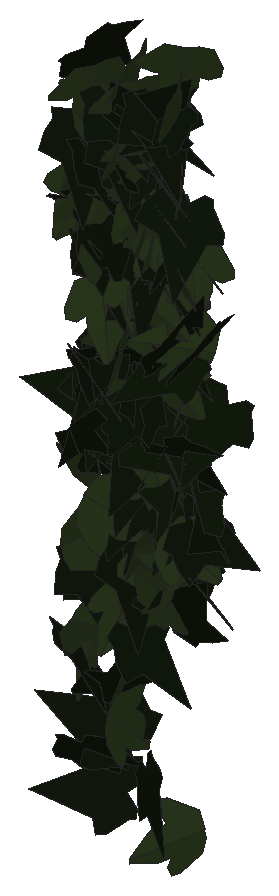
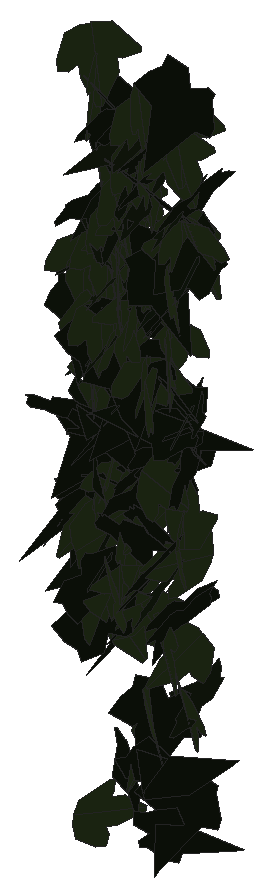
# SketchUp Ruby script. Lengths in inches.
U = 1.inch
M = Sketchup.active_model
def pt(a) = Geom::Point3d.new(a.map { |v| v * U })
def face(e, loops, mat)
  f = e.add_face(loops[0].map { |a| pt(a) })
  loops[1..].each { |l| e.add_face(l.map { |a| pt(a) }).erase! }
  f.material = f.back_material = mat if mat
  f
end
# faces: each face lists its corners as indices into pts; further lists are holes
def faces(e, pts, list, mat = nil) = list.each { |f| face(e, (f[0].is_a?(Array) ? f : [f]).map { |l| l.map { |i| pts[i] } }, mat) }
# xy, xz, yz: faces in a plane at the given z, y or x. An outline is a flat list of corners, or four numbers for a rectangle; further outlines are holes
def ring(l) = l.size == 4 ? [[l[0], l[1]], [l[2], l[1]], [l[2], l[3]], [l[0], l[3]]] : l.each_slice(2).to_a
def flat(e, list, mat, &to3) = list.each { |f| face(e, (f[0].is_a?(Array) ? f : [f]).map { |l| ring(l).map { |u, v| to3.(u, v) } }, mat) }
def xy(e, z, list, mat = nil) = flat(e, list, mat) { |x, y| [x, y, z] }
def xz(e, y, list, mat = nil) = flat(e, list, mat) { |x, z| [x, y, z] }
def yz(e, x, list, mat = nil) = flat(e, list, mat) { |y, z| [x, y, z] }
def lines(e, pts, list) = list.each { |a, b| e.add_line(pt(pts[a]), pt(pts[b])) }
# prism: a flat outline (further loops are holes) pulled along v
def prism(e, loops, v, mat = nil)
  f = face(e, loops, mat); d = Geom::Vector3d.new(v.map { |x| x * U })
  f.pushpull(f.normal.samedirection?(d) ? d.length : -d.length)
end
def box(e, o, s, mat = nil) = prism(e, [[o, [o[0] + s[0], o[1], o[2]], [o[0] + s[0], o[1] + s[1], o[2]], [o[0], o[1] + s[1], o[2]]]], [0, 0, s[2]], mat)
def at(x, y, z, deg = 0) = Geom::Transformation.translation(pt([x, y, z])) * Geom::Transformation.rotation(ORIGIN, Z_AXIS, deg.degrees)
def axes(o, x, y, z) = Geom::Transformation.new([*x, 0, *y, 0, *z, 0, *pt(o).to_a, 1])
def part(name) = M.definitions.add(name)
# library, detail: a bought-in or finely detailed component or shape, given as its bounding box
def library(name, o, s) = part(name).tap { |d| box(d.entities, o, s) }
def detail(e, o, s) = box(e.add_group.entities, o, s)
def put(e, d, t, mat = nil) = e.add_instance(d, t).tap { |i| i.material = mat if mat }
def group(e, t, mat = nil) = e.add_group.tap { |g| g.transformation = t; g.material = mat if mat }.entities
root = M.entities
M.materials.add("efeu1").color = [18, 25, 13]
M.materials.add("efeu2").color = [43, 57, 29]
c1 = part("ivyleaf_10")
p = [[0,0.5,-0.03],[-0.0625,2.02,-0.43],[-0.19,2.01,-0.46],[-0.54,1.05,-0.29],[-0.52,0.625,-0.18],[-0.83,0.76,-0.28],
  [-1.16,0.64,-0.33],[-1.15,0.33,-0.24],[-0.77,-0.39,0.02],[-0.3,-0.51,0.16],[0.04,-0.48,0.23],[-0.02,2.01,-0.4375],
  [-0.06,2.01,-0.43],[0.04,-0.49,0.23],[0.67,-0.49,0.14],[1.38,0.36,-0.2],[1.375,0.51,-0.24],[0.81,0.65,-0.19],
  [0.62,0.59,-0.15],[0.6,1.09,-0.28],[0.5,1.23,-0.31]]
faces(c1.entities,p,[[0,1,2,3,4,5,6,7,8,9,10],[11,12,0,13,14,15,16,17,18,19,20]],"efeu2")
c2 = part("ivyleaf_9")
p = [[1.54,2.16,1.25],[1.36,2.04,1.19],[-0.21,0.99,0.68],[-0.71,1.11,0.82],[-0.85,0.86,0.67],[-0.8,0.17,0.21],
  [-0.9,-0.01,0.1],[-0.67,-0.16,-0.02],[-0.08,-0.08,-0.05],[-0.03,-0.6,-0.4],[0.65,-0.88,-0.66],[0.83,-0.6,-0.49],
  [1.29,-0.42,-0.43],[1.8125,-0.07,-0.26],[1.21,0.44,0.15]]
faces(c2.entities,p,[[0,1,2,3,4,5,6,7,8,9,10,11,12,13,14]],"efeu1")
put(root,c1,axes([534.62,135.42,188.35],[0.65935,-0.44061,0.12588],[0.1096,-0.06254,-0.79297],[0.44494,0.66834,0.00879]))
put(root,c1,axes([534.84,134.72,201.15],[0.75412,-0.21779,-0.249],[-0.2252,0.11603,-0.78355],[0.24231,0.78564,0.04669]))
put(root,c2,axes([534.76,135.05,185.55],[0.67039,0.39495,-0.20021],[-0.17138,-0.10353,-0.77808],[-0.40829,0.69195,-0.00214]))
put(root,c2,axes([534.37,135.18,188.14],[0.29214,-0.6095,0.36994],[0.24797,-0.28798,-0.67028],[0.66848,0.37319,0.08696]))
put(root,c2,axes([535.5,135.61,184.25],[-0.50673,-0.01581,0.6028],[-0.60281,-0.00682,-0.50692],[0.01539,-0.78746,-0.00771]))
put(root,c2,axes([535.57,134.98,195.46],[-0.46793,0.18813,0.62786],[-0.63373,0.06703,-0.49239],[-0.16728,-0.78018,0.1091]))
put(root,c2,axes([534.68,135.07,202.5],[0.04718,-0.829,0.02894],[-0.02015,-0.03012,-0.83005],[0.82926,0.04644,-0.02181]))
put(root,c2,axes([535.57,135.64,185.74],[-0.16714,0.06845,0.8358],[-0.83569,0.05731,-0.17181],[-0.06977,-0.85042,0.0557]))
put(root,c1,axes([535.02,135.42,200.09],[0.28756,-0.76041,-0.04757],[-0.01021,0.04699,-0.81294],[0.76183,0.28765,0.00706]))
put(root,c1,axes([534.85,135.1,192.89],[-0.73914,0.10485,0.29304],[0.28257,-0.09043,0.74509],[0.13045,0.78995,0.0464]))
put(root,c1,axes([535.38,135.08,203.71],[-0.68667,-0.27736,0.36474],[-0.30278,-0.21857,-0.73623],[0.34393,-0.74618,0.08008]))
put(root,c2,axes([534.64,134.71,200.8125],[0.78179,0.14935,0.20417],[0.16207,0.21347,-0.77675],[-0.19422,0.7793,0.17365]))
put(root,c2,axes([534.8,135.32,194.78],[0.10445,-0.27062,-0.74441],[0.57646,-0.48897,0.25864],[-0.54321,-0.57094,0.13134]))
put(root,c2,axes([534.85,134.99,196.34],[0.56446,-0.45809,-0.33124],[-0.257,0.20897,-0.72696],[0.50351,0.62021,0.00028]))
put(root,c1,axes([535.4,135.1,197.8],[0.17744,-0.38074,-0.71286],[-0.30426,0.64467,-0.42006],[0.7487,0.35221,-0.00176]))
put(root,c1,axes([535.18,136,194.66],[-0.01205,-0.56281,0.54498],[0.03984,-0.54478,-0.56172],[0.78241,0.01907,0.03699]))
put(root,c1,axes([534.75,135.48,192.54],[0.21381,-0.30403,0.73736],[0.5785,-0.46643,-0.36006],[0.54907,0.60981,0.09223]))
put(root,c2,axes([534.86,135.24,190.64],[0.22126,-0.70973,-0.26985],[-0.06169,0.26334,-0.7432],[0.75679,0.22897,0.01831]))
put(root,c2,axes([535.15,134.67,205.17],[0.31691,0.72566,0.23951],[0.12455,0.20678,-0.79127],[-0.75395,0.33918,-0.03004]))
put(root,c1,axes([535.1875,134.81,201.23],[-0.1308,-0.81296,-0.08467],[0.09636,0.06981,-0.81916],[0.81166,-0.1393,0.08361]))
put(root,c1,axes([535.28,134.83,204.375],[-0.35242,-0.76911,-0.03582],[0.01252,0.03367,-0.846],[0.76984,-0.35264,-0.00264]))
put(root,c2,axes([534.95,135.07,190.81],[0.0908,-0.72471,-0.26389],[-0.02171,0.2632,-0.7303],[0.77095,0.09277,0.01051]))
put(root,c1,axes([535.18,134.71,201.09],[-0.80741,-0.01746,-0.16808],[0.16765,0.01997,-0.80745],[0.02116,-0.82448,-0.016]))
put(root,c2,axes([534.95,134.81,200.48],[0.67852,-0.34345,-0.31279],[-0.23656,0.22106,-0.75588],[0.39979,0.71369,0.08361]))
put(root,c2,axes([535.55,135.38,200.37],[-0.22617,0.73716,-0.26414],[0.01669,-0.27033,-0.76874],[-0.78287,-0.21873,0.05992]))
put(root,c2,axes([535.1875,135.68,195.46],[-0.32941,-0.71418,0.01216],[-0.00033,-0.01324,-0.78647],[0.71428,-0.32937,0.00525]))
put(root,c1,axes([535.09,134.57,189.33],[-0.2664,-0.34579,-0.60588],[0.35096,0.49407,-0.43629],[0.6029,-0.4404,-0.01374]))
put(root,c1,axes([535.19,134.3125,191.69],[0.0237,-0.15167,0.87928],[-0.02671,0.87908,0.15235],[-0.89187,-0.03036,0.0188]))
put(root,c1,axes([535.58,135.17,189.86],[0.50124,-0.42503,-0.47194],[-0.29702,0.37454,-0.65278],[0.56138,0.57766,0.076]))
put(root,c2,axes([534.85,135.25,195.66],[0.18346,-0.44461,0.62928],[0.37405,-0.51415,-0.47231],[0.67362,0.40658,0.09088]))
put(root,c2,axes([535.06,135.19,199.48],[0.3081,-0.73797,-0.06503],[-0.00691,0.06756,-0.79947],[0.7408,0.30756,0.01959]))
put(root,c2,axes([534.82,135.23,196.13],[0.55414,-0.133,0.56275],[0.5721,0.23954,-0.50673],[-0.08417,0.75258,0.26074]))
put(root,c2,axes([535.53,135.23,196.9375],[-0.70733,-0.01372,-0.3327],[0.33297,-0.03678,-0.70638],[-0.00326,-0.7808,0.03912]))
put(root,c2,axes([535.53,135.0625,187.78],[0.43921,0.647,-0.13895],[-0.0784,-0.11472,-0.78199],[-0.65709,0.44615,0.00042]))
put(root,c2,axes([535.2,135.88,192.2],[0.18454,-0.7603,0.01318],[0.00395,-0.0126,-0.78238],[0.76041,0.18458,0.00087]))
put(root,c2,axes([535.07,134.99,202],[0.46871,-0.68381,0.0131],[0.03688,0.00941,-0.82826],[0.68295,0.4688,0.03573]))
put(root,c1,axes([535.45,135.78,196.91],[0.28905,-0.69765,0.23424],[0.21192,-0.16209,-0.74428],[0.70475,0.33488,0.12773]))
put(root,c2,axes([535.2,135.68,191.3],[0.31404,-0.70545,0.17567],[0.06055,-0.16532,-0.7721],[0.72447,0.31961,-0.01162]))
put(root,c1,axes([535.68,135.51,187.83],[0.36324,-0.67557,-0.0886],[-0.05749,0.06965,-0.76684],[0.67893,0.36735,-0.01753]))
put(root,c1,axes([535.43,134.85,198.39],[0.79984,0.16606,0.22125],[0.21587,0.04862,-0.81689],[-0.17299,0.82845,0.00359]))
put(root,c1,axes([535.83,135.38,197.18],[-0.64268,-0.45043,0.00271],[-0.00221,-0.00157,-0.78481],[0.45043,-0.64269,0.00002]))
put(root,c1,axes([535.77,134.32,200.26],[0.06572,0.58553,0.60075],[-0.10493,0.6036,-0.57682],[-0.8323,-0.02987,0.12015]))
put(root,c1,axes([535.97,134.875,186.68],[-0.11002,0.53422,0.6029],[-0.18627,0.57514,-0.54361],[-0.7837,-0.21169,0.04457]))
put(root,c2,axes([535.36,134.42,194.16],[0.25036,-0.00027,0.79652],[0.77861,0.17616,-0.24467],[-0.16798,0.81615,0.05308]))
put(root,c1,axes([535.87,135.5,196.83],[-0.0549,0.31499,-0.746],[0.03855,-0.74585,-0.31776],[-0.80886,-0.05692,0.03549]))
put(root,c2,axes([535.9,134.56,199.56],[-0.19596,-0.34475,0.75162],[0.58761,0.48542,0.37585],[-0.58181,0.60638,0.12644]))
put(root,c2,axes([535.65,135.13,203.71],[0.2342,-0.74444,-0.2667],[0.0546,0.29271,-0.7691],[0.78889,0.20074,0.1324]))
put(root,c1,axes([536.13,135.04,190.14],[0.47574,0.52141,-0.33208],[-0.24723,-0.22359,-0.70524],[-0.56659,0.53536,0.02889]))
put(root,c1,axes([536.18,135.23,204.83],[0.17272,-0.79658,-0.11877],[-0.01567,0.11813,-0.81503],[0.80523,0.17316,0.00962]))
put(root,c1,axes([536.18,134.96,202.875],[0.19418,-0.7978,-0.16362],[-0.00479,0.16709,-0.82038],[0.81439,0.1912,0.03419]))
put(root,c2,axes([536.8,134.53,195.84],[-0.61517,0.45173,0.46743],[-0.37646,0.27706,-0.76321],[-0.52993,-0.72122,-0.00043]))
put(root,c2,axes([536.33,135.34,197.54],[0.44798,0.52469,-0.43253],[-0.35392,-0.26235,-0.68482],[-0.58062,0.56475,0.08372]))
put(root,c2,axes([536.3,135.27,192.99],[-0.7213,-0.06709,-0.23637],[0.23694,0.0041,-0.72421],[0.06504,-0.75903,0.01699]))
put(root,c2,axes([535.87,135.1,202.79],[0.16429,-0.81077,-0.06081],[-0.02385,0.05721,-0.82716],[0.8127,0.16558,-0.01198]))
put(root,c2,axes([536.81,135.09,202.33],[-0.67465,0.34949,0.34378],[-0.36781,0.02578,-0.74802],[-0.3241,-0.75676,0.13328]))
put(root,c2,axes([536.07,135.6875,193.91],[-0.24356,-0.75318,0.12948],[-0.02391,-0.12832,-0.7914],[0.76385,-0.24417,0.01651]))
put(root,c1,axes([535.97,134.14,193.01],[0.12189,0.57494,0.68034],[0.13848,0.6661,-0.58771],[-0.87991,0.18448,0.00175]))
put(root,c2,axes([535.97,135.1,196.61],[0.69878,0.39802,0.06626],[0.05292,0.04097,-0.80413],[-0.40001,0.70071,0.00938]))
put(root,c1,axes([536.4,134.99,204.26],[-0.3645,-0.74114,0.00565],[-0.00315,-0.00475,-0.82592],[0.74115,-0.36451,-0.00073]))
put(root,c2,axes([536.32,135.84,192.85],[-0.63495,-0.31036,-0.28574],[0.28803,0.05834,-0.70339],[0.30824,-0.69383,0.06867]))
put(root,c2,axes([536.24,135.4,194.29],[-0.13244,-0.68712,0.35712],[-0.07492,-0.34923,-0.69973],[0.77075,-0.15202,-0.00666]))
put(root,c1,axes([536.35,135.26,198.91],[-0.30631,0.64826,-0.3505],[-0.0139,-0.38458,-0.69916],[-0.73682,-0.26224,0.1589]))
put(root,c1,axes([536.27,135.28,198.92],[0.49155,0.62875,0.00723],[0.00104,0.00836,-0.79808],[-0.62879,0.49153,0.00433]))
put(root,c1,axes([536.58,135.08,202.99],[-0.14124,-0.81188,0.10003],[-0.02726,-0.09678,-0.82401],[0.81756,-0.14349,-0.01019]))
put(root,c2,axes([536.14,135.17,190.97],[0.12675,-0.77791,0.17103],[0.05606,-0.16404,-0.78766],[0.79451,0.13567,0.02829]))
put(root,c2,axes([536.02,135.18,202.03],[0.59458,-0.57068,0.06103],[0.10893,0.02594,-0.81878],[0.5635,0.59714,0.09388]))
put(root,c1,axes([536.44,135.1875,191.1],[0.2707,0.72972,0.18984],[0.06971,0.17662,-0.7783],[-0.75077,0.27951,-0.00382]))
put(root,c1,axes([536.74,135.22,202.02],[-0.25605,-0.78178,0.04635],[-0.00725,-0.0464,-0.82261],[0.78312,-0.25604,0.00754]))
put(root,c1,axes([536.67,135.17,200.75],[0.39345,-0.72155,-0.09482],[0.01599,0.11633,-0.81892],[0.72757,0.38763,0.06927]))
put(root,c1,axes([536.74,135.03,192.05],[0.12936,-0.71454,-0.36284],[0.00732,0.36857,-0.72323],[0.80136,0.11198,0.06518]))
put(root,c1,axes([537.08,135.46,190.1],[-0.51209,-0.35145,0.50491],[-0.3983,-0.31126,-0.62062],[0.46884,-0.6483,0.02425]))
put(root,c2,axes([536.54,134.98,196.08],[0.47358,-0.22128,-0.60084],[-0.28342,0.59768,-0.44351],[0.57415,0.47756,0.27666]))
put(root,c1,axes([536.67,134.77,201.24],[0.22358,0.77697,0.06202],[-0.03068,0.07325,-0.80698],[-0.77884,0.22016,0.0496]))
put(root,c1,axes([536.68,135.5,190.25],[0.59652,-0.54701,0.10178],[-0.05942,0.08573,0.80903],[-0.55322,-0.59904,0.02285]))
put(root,c2,axes([536.54,135.49,198.76],[-0.33373,-0.51834,-0.50701],[0.38098,0.34953,-0.60811],[0.61692,-0.49625,0.10126]))
put(root,c1,axes([536.96,135.37,199.86],[0.47548,-0.56022,-0.32375],[-0.14223,0.30144,-0.73051],[0.63122,0.48992,0.07927]))
put(root,c2,axes([536.39,135.02,203.68],[0.70682,-0.4366,-0.08092],[0.08441,0.28147,-0.78129],[0.43593,0.65339,0.28249]))
put(root,c2,axes([536.78,135.12,199.92],[-0.60141,-0.14342,-0.53726],[0.5297,0.09306,-0.61779],[0.16921,-0.80105,0.02442]))
put(root,c1,axes([536.85,135.36,198.08],[0.74408,-0.28657,-0.11983],[0.00017,0.31143,-0.74374],[0.31062,0.68631,0.28745]))
put(root,c1,axes([536.97,135.21,197.76],[-0.25013,0.76244,-0.04402],[-0.10858,-0.08136,-0.7921],[-0.75596,-0.24059,0.12833]))
put(root,c1,axes([536.8125,135.26,199.93],[0.33824,-0.71561,0.13946],[0.24483,-0.03333,-0.76479],[0.68673,0.36434,0.20396]))
put(root,c1,axes([537.12,135.46,190.25],[-0.26786,-0.50231,-0.56287],[-0.27471,-0.49135,0.56921],[-0.70262,0.3836,-0.00796]))
put(root,c1,axes([536.9,135.15,193.76],[-0.55826,-0.46717,-0.23901],[0.31045,-0.01268,-0.70034],[0.42307,-0.60714,0.19854]))
put(root,c1,axes([537.18,135.6,198.46],[-0.44689,-0.6571,0.00396],[-0.01023,0.00216,-0.79461],[0.65703,-0.4469,-0.00967]))
put(root,c1,axes([537.18,135.35,200.43],[-0.59415,-0.54419,-0.00207],[-0.00044,0.00355,-0.8057],[0.5442,-0.59415,-0.00291]))
put(root,c1,axes([537.16,135.18,201.08],[-0.21659,-0.79568,0.03401],[0.00997,-0.03795,-0.8244],[0.79634,-0.21593,0.01957]))
put(root,c2,axes([536.75,134.51,189.625],[0.44554,-0.55438,-0.39868],[-0.11042,0.41128,-0.6953],[0.67386,0.43393,0.14966]))
put(root,c2,axes([536.73,135.44,199.84],[0.43806,-0.68165,-0.06351],[0.01579,0.08544,-0.8081],[0.68442,0.43431,0.05929]))
put(root,c2,axes([537.34,136.05,191.17],[-0.012,-0.02168,-0.77136],[0.12578,-0.76119,0.01944],[-0.76135,-0.12541,0.01537]))
put(root,c2,axes([536.78,134.97,185.48],[-0.12587,-0.08121,-0.76685],[0.77097,-0.02924,-0.12345],[-0.01587,-0.77656,0.08484]))
put(root,c2,axes([536.8,134.79,203.44],[-0.27642,-0.1586,0.77641],[0.74387,-0.33539,0.19633],[0.27317,0.75282,0.25103]))
put(root,c2,axes([536.92,134.95,202.3125],[0.7595,-0.24942,-0.17916],[-0.16331,0.07673,-0.79912],[0.26008,0.77656,0.02141]))
put(root,c2,axes([537.67,134.96,200.37],[-0.54927,0.60141,-0.01408],[0.01065,-0.00935,-0.81448],[-0.60148,-0.54937,-0.00156]))
put(root,c1,axes([537.3,135.16,194.24],[-0.55741,0.54017,0.0108],[-0.00872,0.00652,-0.7762],[-0.54021,-0.55747,0.00139]))
put(root,c2,axes([536.89,135.41,197.97],[0.51506,-0.61224,-0.09127],[0.00715,0.12461,-0.79554],[0.61897,0.50802,0.08514]))
put(root,c1,axes([537.1875,135.16,200.22],[0.38768,0.70478,0.03202],[0.01904,0.02608,-0.80436],[-0.70525,0.38813,-0.00411]))
put(root,c2,axes([537.91,135.36,194.87],[-0.65386,-0.00067,0.41071],[-0.41046,-0.02625,-0.6535],[0.01453,-0.77171,0.02187]))
put(root,c2,axes([537.11,135.03,204.08],[0.0554,-0.78877,-0.26566],[-0.01652,0.26515,-0.79071],[0.83214,0.05777,0.00198]))
put(root,c1,axes([536.85,134.82,198.79],[-0.28131,-0.02452,-0.75855],[0.70365,-0.31156,-0.25088],[-0.28439,-0.74664,0.1296]))
put(root,c1,axes([537.17,135.2,196.69],[-0.68935,-0.16399,-0.41324],[0.41581,0.03205,-0.70636],[0.15736,-0.80309,0.0562]))
put(root,c2,axes([536.98,135.64,189.61],[0.82613,0.079,-0.10325],[0.08781,0.15072,0.8179],[0.09587,-0.8188,0.14059]))
put(root,c1,axes([537.71,135.48,191.77],[-0.12254,-0.1424,-0.78255],[-0.40287,-0.67159,0.1853],[-0.68582,0.41995,0.03097]))
put(root,c2,axes([537.94,134.92,204.41],[-0.78988,0.28737,0.03998],[-0.04529,-0.0076,-0.84022],[-0.28658,-0.79085,0.0226]))
put(root,c1,axes([537.69,135.4,183.92],[-0.16005,-0.02137,0.78363],[-0.12328,-0.78916,-0.0467],[0.77417,-0.13009,0.15457]))
put(root,c2,axes([537.98,135.05,197.48],[-0.765,-0.07871,0.18196],[-0.17628,-0.06188,-0.76787],[0.09073,-0.7839,0.04235]))
put(root,c2,axes([537.85,134.67,193.46],[-0.04655,0.20816,0.79895],[-0.06491,0.79682,-0.21138],[-0.82307,-0.07462,-0.02851]))
put(root,c2,axes([537.19,135.11,201.02],[0.74961,-0.31422,-0.06319],[-0.06123,0.01738,-0.81277],[0.31461,0.75207,-0.00762]))
put(root,c1,axes([537.55,135.08,202.34],[0.64081,-0.52438,0.07588],[0.13255,0.04337,-0.81971],[0.513,0.64383,0.11702]))
put(root,c1,axes([537.94,135,196.92],[0.25869,-0.50635,-0.65736],[-0.27444,0.5976,-0.56832],[0.78307,0.37672,0.01798]))
put(root,c2,axes([537.99,135.01,195.86],[-0.55514,0.56396,-0.37891],[0.24057,-0.29445,-0.79071],[-0.63542,-0.60419,0.03168]))
put(root,c2,axes([537.52,134.84,194.83],[0.70419,0.3322,0.01886],[0.0174,0.00732,-0.77862],[-0.33228,0.70441,-0.00081]))
put(root,c1,axes([538.05,135.27,197.5625],[0.08191,0.3062,0.83194],[-0.25615,-0.79167,0.31659],[0.84868,-0.2685,0.01526]))
put(root,c2,axes([537.88,135.48,193.37],[-0.61069,-0.44917,-0.07114],[0.06923,0.02589,-0.75783],[0.44947,-0.61428,0.02008]))
put(root,c1,axes([537.99,134.92,205.76],[-0.61972,-0.55124,0.12887],[-0.09273,-0.08965,-0.82939],[0.55846,-0.6266,0.00529]))
put(root,c1,axes([538.12,134.5,200.17],[-0.53788,0.34717,0.51128],[-0.41102,0.30521,-0.63966],[-0.46152,-0.67644,-0.02621]))
put(root,c1,axes([537.89,134.75,204.8],[0.13743,-0.66064,-0.502],[-0.0089,0.50763,-0.6705],[0.82968,0.11488,0.07596]))
put(root,c2,axes([537.53,134.91,197.29],[0.41595,0.67466,0.34934],[-0.17093,-0.30496,0.79247],[0.74027,-0.44951,-0.0133]))
put(root,c2,axes([537.45,135.22,191.6],[0.68626,-0.32844,0.01237],[0.01566,0.00408,-0.76074],[0.3283,0.68636,0.01044]))
put(root,c1,axes([537.92,135.37,200],[-0.68359,-0.44398,0.00443],[0.12716,-0.20357,-0.77899],[0.42541,-0.65259,0.23998]))
put(root,c2,axes([537.86,135.17,201.47],[-0.15313,-0.81155,0.03216],[-0.00645,-0.03151,-0.82587],[0.81216,-0.15327,-0.0005]))
put(root,c1,axes([537.88,134.76,192.37],[0.19537,0.55454,0.53094],[0.15785,0.50714,-0.58777],[-0.75133,0.25074,0.01458]))
put(root,c2,axes([538.04,136.1875,192.52],[-0.11178,-0.41339,0.63331],[-0.02147,-0.6382,-0.42037],[0.75598,-0.07925,0.08171]))
put(root,c2,axes([538.03,135.02,192.82],[0.38738,-0.26974,-0.66955],[-0.22332,0.67781,-0.40227],[0.68643,0.37274,0.24698]))
put(root,c2,axes([538.5625,134.61,197.99],[-0.06736,0.75977,0.21306],[-0.00064,0.21378,-0.76255],[-0.78908,-0.06503,-0.01757]))
put(root,c2,axes([538.375,135.99,195.75],[-0.65078,-0.41805,-0.11858],[0.19009,-0.08187,-0.75465],[0.39075,-0.65641,0.16964]))
